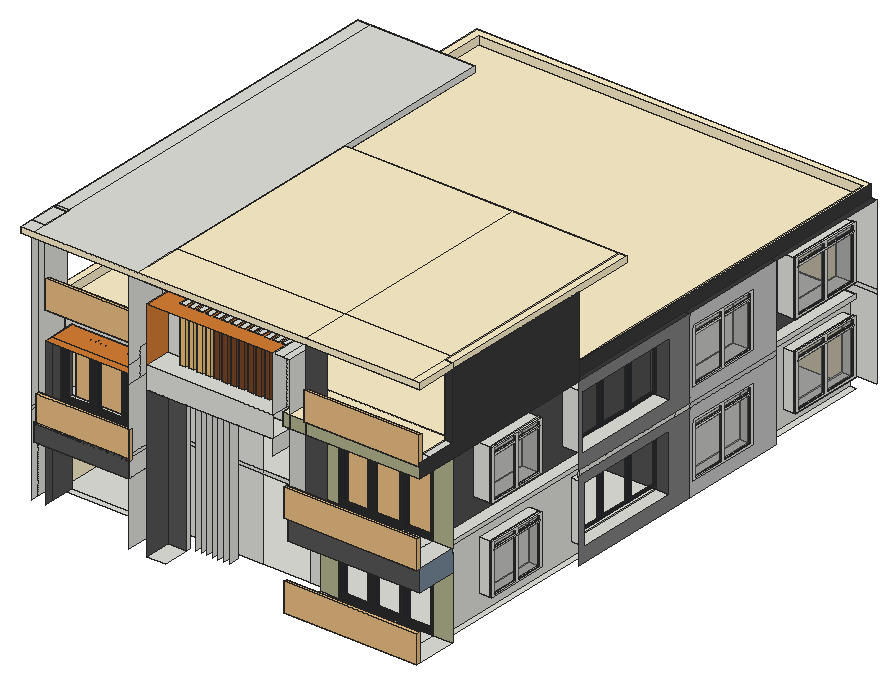
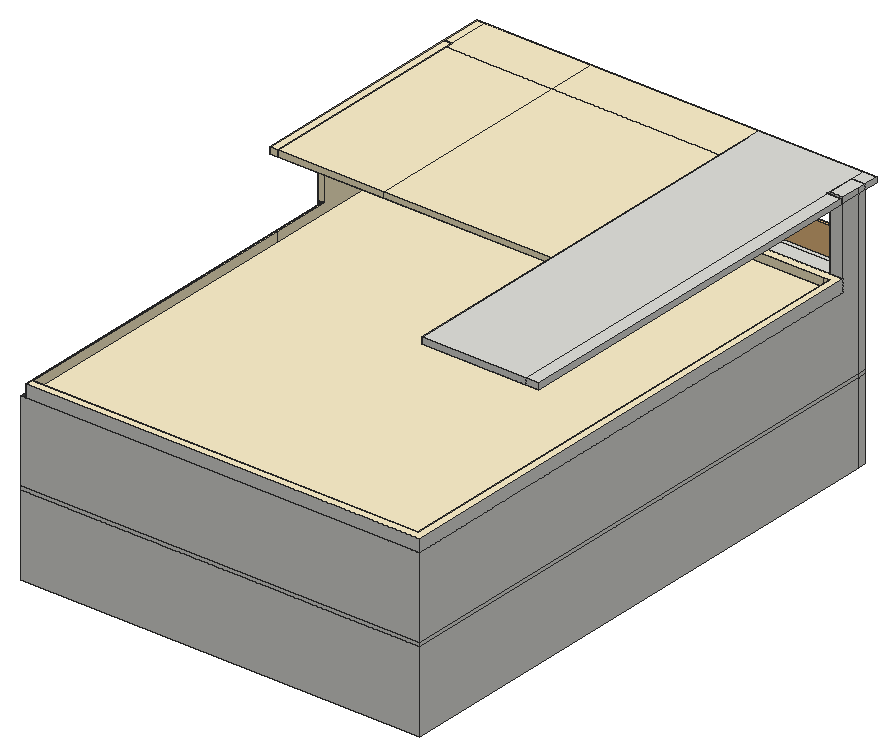
# SketchUp Ruby script. Lengths in inches.
U = 1.inch
M = Sketchup.active_model
def pt(a) = Geom::Point3d.new(a.map { |v| v * U })
def face(e, loops, mat)
  f = e.add_face(loops[0].map { |a| pt(a) })
  loops[1..].each { |l| e.add_face(l.map { |a| pt(a) }).erase! }
  f.material = f.back_material = mat if mat
  f
end
# faces: each face lists its corners as indices into pts; further lists are holes
def faces(e, pts, list, mat = nil) = list.each { |f| face(e, (f[0].is_a?(Array) ? f : [f]).map { |l| l.map { |i| pts[i] } }, mat) }
# xy, xz, yz: faces in a plane at the given z, y or x. An outline is a flat list of corners, or four numbers for a rectangle; further outlines are holes
def ring(l) = l.size == 4 ? [[l[0], l[1]], [l[2], l[1]], [l[2], l[3]], [l[0], l[3]]] : l.each_slice(2).to_a
def flat(e, list, mat, &to3) = list.each { |f| face(e, (f[0].is_a?(Array) ? f : [f]).map { |l| ring(l).map { |u, v| to3.(u, v) } }, mat) }
def xy(e, z, list, mat = nil) = flat(e, list, mat) { |x, y| [x, y, z] }
def xz(e, y, list, mat = nil) = flat(e, list, mat) { |x, z| [x, y, z] }
def yz(e, x, list, mat = nil) = flat(e, list, mat) { |y, z| [x, y, z] }
def lines(e, pts, list) = list.each { |a, b| e.add_line(pt(pts[a]), pt(pts[b])) }
# prism: a flat outline (further loops are holes) pulled along v
def prism(e, loops, v, mat = nil)
  f = face(e, loops, mat); d = Geom::Vector3d.new(v.map { |x| x * U })
  f.pushpull(f.normal.samedirection?(d) ? d.length : -d.length)
end
def box(e, o, s, mat = nil) = prism(e, [[o, [o[0] + s[0], o[1], o[2]], [o[0] + s[0], o[1] + s[1], o[2]], [o[0], o[1] + s[1], o[2]]]], [0, 0, s[2]], mat)
def at(x, y, z, deg = 0) = Geom::Transformation.translation(pt([x, y, z])) * Geom::Transformation.rotation(ORIGIN, Z_AXIS, deg.degrees)
def axes(o, x, y, z) = Geom::Transformation.new([*x, 0, *y, 0, *z, 0, *pt(o).to_a, 1])
def part(name) = M.definitions.add(name)
# library, detail: a bought-in or finely detailed component or shape, given as its bounding box
def library(name, o, s) = part(name).tap { |d| box(d.entities, o, s) }
def detail(e, o, s) = box(e.add_group.entities, o, s)
def put(e, d, t, mat = nil) = e.add_instance(d, t).tap { |i| i.material = mat if mat }
def group(e, t, mat = nil) = e.add_group.tap { |g| g.transformation = t; g.material = mat if mat }.entities
root = M.entities
M.materials.add("Wine2").color = [0, 0, 0]
M.materials["Wine2"].alpha = 0
M.materials.add("[0110_LightSlateGray]").color = [119, 136, 153]
M.materials.add("[0130_Gainsboro]").color = [39, 45, 50]
M.materials.add("[0133_Gray]").color = [128, 128, 128]
M.materials.add("[0135_DarkGray]1").color = [81, 81, 81]
M.materials.add("[Color D01]").color = [255, 242, 204]
M.materials.add("[Color E01]").color = [178, 178, 142]
M.materials.add("[Color M02]").color = [198, 198, 198]
M.materials.add("[Color M06]").color = [86, 86, 86]
M.materials.add("[Color M07]").color = [58, 58, 58]
M.materials.add("[Translucent Glass Gray]").color = [128, 128, 128]
M.materials["[Translucent Glass Gray]"].alpha = 0.5
M.materials.add("[Wood Bamboo]").color = [214, 127, 52]
M.materials.add("[Wood OSB]").color = [240, 195, 122]
M.materials.add("[Wood Veneer 01]").color = [120, 70, 37]
c1 = part("Framed glazing panel")
xy(c1.entities,0,[[0,-0.98,43.07,0],[0,0,43.07,1.4]],"[0130_Gainsboro]")
xy(c1.entities,0.3,[[0.3,-1.43,42.77,-0.98]],"[0130_Gainsboro]")
xy(c1.entities,2.95,[[2.95,-1.43,40.12,-0.63],[2.95,-0.63,40.12,0],[2.95,0,40.12,0.64],[2.95,0.64,40.12,1.4]],"[0130_Gainsboro]")
xy(c1.entities,3.54,[[3.54,-0.63,39.53,0],[3.54,0,39.53,0.64]],"[0130_Gainsboro]")
xy(c1.entities,111.8125,[[3.54,-0.63,39.53,0],[3.54,0,39.53,0.64]],"[0130_Gainsboro]")
xy(c1.entities,112.4,[[2.95,-1.43,40.12,-0.63],[2.95,-0.63,40.12,0],[2.95,0,40.12,0.64],[2.95,0.64,40.12,1.4]],"[0130_Gainsboro]")
xy(c1.entities,115.05,[[0.3,-1.43,42.77,-0.98]],"[0130_Gainsboro]")
xy(c1.entities,115.35,[[0,-0.98,43.07,0],[0,0,43.07,1.4]],"[0130_Gainsboro]")
xz(c1.entities,-1.43,[[[0.3,0.3,42.77,115.05],[2.95,2.95,40.12,112.4]]],"[0130_Gainsboro]")
xz(c1.entities,-0.98,[[[0,0,43.07,115.35],[0.3,0.3,42.77,115.05]]],"[0130_Gainsboro]")
xz(c1.entities,-0.63,[[[2.95,2.95,40.12,112.4],[3.54,3.54,39.53,111.8125]]],"[0130_Gainsboro]")
xz(c1.entities,0,[[3.54,3.54,39.53,111.8125]],"Wine2")
xz(c1.entities,0,[[[0,0,43.07,115.35],[2.95,2.95,40.12,112.4]],[[2.95,2.95,40.12,112.4],[3.54,3.54,39.53,111.8125]]],"[0130_Gainsboro]")
xz(c1.entities,0.64,[[[2.95,2.95,40.12,112.4],[3.54,3.54,39.53,111.8125]]],"[0130_Gainsboro]")
xz(c1.entities,1.4,[[[0,0,43.07,115.35],[2.95,2.95,40.12,112.4]]],"[0130_Gainsboro]")
yz(c1.entities,0,[[-0.98,0,0,115.35],[0,0,1.4,115.35]],"[0130_Gainsboro]")
yz(c1.entities,0.3,[[-1.43,0.3,-0.98,115.05]],"[0130_Gainsboro]")
yz(c1.entities,2.95,[[-1.43,2.95,-0.63,112.4],[-0.63,2.95,0,112.4],[0,2.95,0.64,112.4],[0.64,2.95,1.4,112.4]],"[0130_Gainsboro]")
yz(c1.entities,3.54,[[-0.63,3.54,0,111.8125],[0,3.54,0.64,111.8125]],"[0130_Gainsboro]")
yz(c1.entities,39.53,[[-0.63,3.54,0,111.8125],[0,3.54,0.64,111.8125]],"[0130_Gainsboro]")
yz(c1.entities,40.12,[[-1.43,2.95,-0.63,112.4],[-0.63,2.95,0,112.4],[0,2.95,0.64,112.4],[0.64,2.95,1.4,112.4]],"[0130_Gainsboro]")
yz(c1.entities,42.77,[[-1.43,0.3,-0.98,115.05]],"[0130_Gainsboro]")
yz(c1.entities,43.07,[[-0.98,0,0,115.35],[0,0,1.4,115.35]],"[0130_Gainsboro]")
c2 = part("Glazing assembly")
put(c2.entities,c1,axes([90.57,1.43,0],[1.05148,0,0],[0,1,0],[0,0,1]))
put(c2.entities,c1,axes([0,1.43,0],[1.05148,0,0],[0,1,0],[0,0,1]))
put(c2.entities,c1,axes([45.29,1.43,0],[1.05148,0,0],[0,1,0],[0,0,1]))
c3 = library("Glass Railing",[0,0,0],[139.5,4.76,42])
c4 = part("Group\#3")
xy(c4.entities,0,[[0,0,32.48,1.97]])
xy(c4.entities,0.98,[[0.98,0,31.5,0.98],[0.98,0.98,31.5,1.97]])
xy(c4.entities,8.86,[[0.98,0,31.5,0.98],[0.98,0.98,31.5,1.97]])
xy(c4.entities,9.84,[[0,0,32.48,1.97]])
xz(c4.entities,0,[[[0,0,32.48,9.84],[0.98,0.98,31.5,8.86]]])
xz(c4.entities,0.98,[[0.98,0.98,31.5,8.86]],"[Translucent Glass Gray]")
xz(c4.entities,1.97,[[[0,0,32.48,9.84],[0.98,0.98,31.5,8.86]]])
yz(c4.entities,0,[[0,0,1.97,9.84]])
yz(c4.entities,0.98,[[0,0.98,0.98,8.86],[0.98,0.98,1.97,8.86]])
yz(c4.entities,31.5,[[0,0.98,0.98,8.86],[0.98,0.98,1.97,8.86]])
yz(c4.entities,32.48,[[0,0,1.97,9.84]])
c5 = part("Group\#4")
xy(c5.entities,0,[[0,0,32.48,1.97]])
xy(c5.entities,0.98,[[0.98,0,31.5,0.98],[0.98,0.98,31.5,1.97]])
xy(c5.entities,71.85,[[0.98,0,31.5,0.98],[0.98,0.98,31.5,1.97]])
xy(c5.entities,72.83,[[0,0,32.48,1.97]])
xz(c5.entities,0,[[[0,0,32.48,72.83],[0.98,0.98,31.5,71.85]]])
xz(c5.entities,0.98,[[0.98,0.98,31.5,71.85]],"[Translucent Glass Gray]")
xz(c5.entities,1.97,[[[0,0,32.48,72.83],[0.98,0.98,31.5,71.85]]])
yz(c5.entities,0,[[0,0,1.97,72.83]])
yz(c5.entities,0.98,[[0,0.98,0.98,71.85],[0.98,0.98,1.97,71.85]])
yz(c5.entities,31.5,[[0,0.98,0.98,71.85],[0.98,0.98,1.97,71.85]])
yz(c5.entities,32.48,[[0,0,1.97,72.83]])
c6 = part("FIXED+GLASS+WINDOW+WITH+TRANSOM")
g1 = group(c6.entities,at(0,0,0))
xy(g1,0,[[0,0,70.86,3.9375]])
xy(g1,1.97,[[1.97,0,34.45,0.98],[36.42,0,68.9,3.9375],[1.97,2.95,34.45,3.9375]])
xy(g1,86.61,[[1.97,0,34.45,3.9375],[34.45,0,36.42,3.9375],[36.42,0,68.9,3.9375]])
xy(g1,88.58,[[0,0,70.86,3.9375]])
xz(g1,0,[[[0,0,70.86,88.58],[1.97,1.97,34.45,86.61],[36.42,1.97,68.9,86.61]]])
xz(g1,3.9375,[[[0,0,70.86,88.58],[1.97,1.97,34.45,86.61],[36.42,1.97,68.9,86.61]]])
yz(g1,0,[[0,0,3.9375,88.58]])
yz(g1,1.97,[[0,1.97,3.9375,74.8],[0,76.77,3.9375,86.61]])
yz(g1,34.45,[[0,1.97,3.9375,86.61]])
yz(g1,36.42,[[0,1.97,3.9375,86.61]])
yz(g1,68.9,[[0,1.97,3.9375,86.61]])
yz(g1,70.86,[[0,0,3.9375,88.58]])
g2 = group(g1,at(1.97,0,74.8))
box(g2,[0,0,0],[66.93,3.9375,1.97])
put(g1,c4,at(1.97,0.98,76.77))
put(g1,c4,at(36.42,0.98,76.77))
put(g1,c5,at(1.97,0.98,1.97))
put(g1,c5,at(36.42,0.98,1.97))
c7 = library("Group5_1",[-7.56,-66.38,0.11],[6.33,135.04,120.95])
xy(root,1007.625,[[326.68,240.0625,354.04,279.375],[536.21,240.3125,563.32,301.625],[563.32,240.3125,704.2,310.82],[704.2,240.3125,733.4375,301.625],[157.82,301.625,298.7,310.82],
  [146.57,310.82,713.5,1067.8],[713.5,310.82,721.74,1067.8]])
xy(root,1027.38,[[713.5,750.25,733.4375,861.32]])
xy(root,1029.41,[[631.25,546.17,713.5,704.54],[713.5,546.17,733.4375,704.54]])
xy(root,1032.83,[[713.5,942.08,733.4375,1053.14]])
xy(root,1036.03,[[713.5,375.23,733.4375,467.6]])
xy(root,1101.6875,[[563.32,301.625,704.2,310.82]])
xy(root,1101.6875,[[157.82,240.3125,298.7,273.3125],[536.21,240.3125,733.4375,301.625],[157.82,273.3125,298.7,310.82]],"[Wood Bamboo]")
xy(root,1108.63,[[713.5,750.25,733.4375,861.32]])
xy(root,1110.53,[[713.5,375.23,733.4375,467.6]])
xy(root,1114.08,[[713.5,942.08,733.4375,1053.14]])
xy(root,1114.73,[[631.25,546.17,713.5,704.54],[713.5,546.17,733.4375,704.54]])
xy(root,1127.625,[[157.82,240.3125,298.7,273.3125],[157.82,273.3125,298.7,301.625],[713.5,310.82,721.74,1067.8]])
xy(root,1127.625,[[146.57,310.82,713.5,1067.8]],"[Color D01]")
xy(root,1133.625,[[539.29,240.0625,563.32,240.3125],[536.21,240.3125,539.29,240.3125,539.29,279.375,563.32,279.375,563.32,301.625,536.21,301.625],[539.29,240.3125,563.32,279.375],[563.32,240.3125,704.2,310.82],[704.2,240.3125,733.4375,301.625],
  [157.82,301.625,298.7,310.82],[146.57,310.82,704.2,1067.8],[704.2,310.82,721.74,1067.8]])
xy(root,1153.38,[[704.2,750.25,733.4375,861.32]])
xy(root,1155.17,[[631.25,541.94,733.4375,706.32]])
xy(root,1158.83,[[704.2,942.08,733.4375,1053.14]])
xy(root,1162.03,[[704.2,375.23,733.4375,467.6]])
xy(root,1208.73,[[442.42,279.375,514.85,310.82]])
xy(root,1227.6875,[[563.32,301.625,704.2,310.82]])
xy(root,1227.6875,[[157.82,261.5,298.7,273.3125],[157.82,273.3125,298.7,310.82]],"[Wood Bamboo]")
xy(root,1230.97,[[326.68,240.0625,354.04,279.375],[354.04,240.0625,354.04,285.875,360.09,285.875,360.09,301.625,362.47,301.625,362.47,285.875,368.53,285.875,368.53,301.625,370.91,301.625,370.91,285.875,376.96,285.875,376.96,301.625,379.35,301.625,379.35,285.875,385.4,285.875,385.4,301.625,387.79,301.625,387.79,285.875,393.84,285.875,393.84,301.625,396.22,301.625,396.22,285.875,402.28,285.875,402.28,301.625,404.66,301.625,404.66,285.875,410.71,285.875,410.71,301.625,413.1,301.625,413.1,285.875,419.15,285.875,419.15,301.625,423.66,301.625,423.66,240.0625],[423.66,240.0625,514.85,279.375]])
xy(root,1234.63,[[704.2,750.25,733.4375,861.32]])
xy(root,1236.53,[[704.2,375.23,733.4375,467.6]])
xy(root,1237.73,[[631.25,541.94,733.4375,706.32]])
xy(root,1240.08,[[704.2,942.08,733.4375,1053.14]])
xy(root,1253.625,[[529.32,240.3125,536.21,301.625],[536.21,240.3125,733.4375,301.625],[[137.375,301.625,733.4375,301.625,733.4375,537.75,725.5,537.75,725.5,1091.875,137.375,1091.875],[146.57,310.82,704.2,1067.8]]])
xy(root,1253.625,[[725.5,537.75,733.4375,744.22],[725.5,744.22,733.4375,904.3],[725.5,904.3,733.4375,1091.875]],"[Color M07]")
xy(root,1259.625,[[148.92,313.17,721.89,1080.33]],"[Color D01]")
xy(root,1263.23,[[326.68,240.0625,514.85,240.0625,514.85,264.875,507.3125,264.875,507.3125,279.375,503.22,279.375,503.22,264.875,494.6875,264.875,494.6875,279.375,490.59,279.375,490.59,264.875,482.0625,264.875,482.0625,279.375,477.97,279.375,477.97,264.875,469.4375,264.875,469.4375,279.375,465.34,279.375,465.34,264.875,456.8125,264.875,456.8125,279.375,452.72,279.375,452.72,264.875,444.1875,264.875,444.1875,279.375,440.09,279.375,440.09,264.875,431.5625,264.875,431.5625,279.375,427.47,279.375,427.47,264.875,418.9375,264.875,418.9375,279.375,414.84,279.375,414.84,264.875,406.3125,264.875,406.3125,279.375,402.22,279.375,402.22,264.875,393.6875,264.875,393.6875,279.375,389.59,279.375,389.59,264.875,381.0625,264.875,381.0625,279.375,376.97,279.375,376.97,264.875,368.4375,264.875,368.4375,279.375,364.34,279.375,364.34,264.875,355.8125,264.875,355.8125,279.375,326.68,279.375]])
xy(root,1269.0625,[[157.51,261.5,298.7,273.3125],[157.51,273.3125,298.7,301.625]])
xy(root,1272.5,[[529.32,240.3125,721.89,240.3125,721.89,313.17,148.92,313.17,148.92,1080.33,721.89,1080.33,721.89,537.75,725.5,537.75,725.5,1091.875,137.375,1091.875,137.375,301.625,529.32,301.625]],"[Color D01]")
xy(root,1275.0625,[[721.89,240.3125,733.4375,258.53],[721.89,258.53,733.4375,301.625]])
xy(root,1345.48,[[514.85,240.0625,529.32,279.375],[529.32,240.0625,539.29,279.375],[355.8125,264.875,364.34,279.375],[368.4375,264.875,376.97,279.375],[381.0625,264.875,389.59,279.375],
  [393.6875,264.875,402.22,279.375],[406.3125,264.875,414.84,279.375],[418.9375,264.875,427.47,279.375],[431.5625,264.875,440.09,279.375],[444.1875,264.875,452.72,279.375],
  [456.8125,264.875,465.34,279.375],[469.4375,264.875,477.97,279.375],[482.0625,264.875,490.59,279.375],[494.6875,264.875,503.22,279.375],[507.3125,264.875,514.85,279.375]])
xy(root,1345.48,[[326.68,240.0625,326.68,279.375,355.8125,279.375,355.8125,264.875,364.34,264.875,364.34,279.375,368.4375,279.375,368.4375,264.875,376.97,264.875,376.97,279.375,381.0625,279.375,381.0625,264.875,389.59,264.875,389.59,279.375,393.6875,279.375,393.6875,264.875,402.22,264.875,402.22,279.375,406.3125,279.375,406.3125,264.875,414.84,264.875,414.84,279.375,418.9375,279.375,418.9375,264.875,427.47,264.875,427.47,279.375,431.5625,279.375,431.5625,264.875,440.09,264.875,440.09,279.375,444.1875,279.375,444.1875,264.875,452.72,264.875,452.72,279.375,456.8125,279.375,456.8125,264.875,465.34,264.875,465.34,279.375,469.4375,279.375,469.4375,264.875,477.97,264.875,477.97,279.375,482.0625,279.375,482.0625,264.875,490.59,264.875,490.59,279.375,494.6875,279.375,494.6875,264.875,503.22,264.875,503.22,279.375,507.3125,279.375,507.3125,264.875,514.85,264.875,514.85,240.0625]],"[Wood Bamboo]")
xy(root,1373.625,[[298.7,240.0625,312.6875,261.5],[312.6875,240.0625,312.6875,301.625,529.32,301.625,529.32,279.375,326.68,279.375,326.68,240.0625],[326.68,240.0625,563.32,279.375],[137.375,261.5,157.51,301.625],[298.7,261.5,312.6875,301.625],
  [298.7,301.625,312.6875,306.6875]])
xy(root,1373.625,[[721.89,301.625,733.4375,537.75],[721.89,537.75,733.4375,626.85]],"[Color D01]")
xy(root,1373.625,[[137.375,240.0625,137.375,261.5,157.51,261.5,157.51,306.6875,137.375,306.6875,137.375,869,312.6875,869,312.6875,306.6875,298.7,306.6875,298.7,240.0625],[563.32,240.0625,563.32,279.375,529.32,279.375,529.32,301.625,312.6875,301.625,312.6875,626.85,721.89,626.85,721.89,301.625,733.4375,301.625,733.4375,240.0625]],"[Color E01]")
xy(root,1382.3125,[[137.375,240.0625,157.51,261.5],[157.51,240.0625,312.6875,869],[137.375,261.5,157.51,301.625],[137.375,306.6875,157.51,869]])
xy(root,1382.3125,[[312.6875,240.0625,563.32,313.17],[563.32,240.0625,721.89,313.17],[721.89,240.0625,733.4375,301.625],[721.89,301.625,733.4375,626.85],[312.6875,313.17,563.32,626.85],
  [563.32,313.17,721.89,626.85]],"[Color D01]")
xz(root,240.0625,[[326.68,1230.97,514.85,1263.23]])
xz(root,240.0625,[[137.375,1373.625,733.4375,1382.3125]],"[Color D01]")
xz(root,240.3125,[[529.32,1253.625,733.4375,1253.625,733.4375,1275.0625,721.89,1275.0625,721.89,1272.5,529.32,1272.5]],"[Color E01]")
xz(root,240.3125,[[157.82,1101.6875,298.7,1127.625],[536.21,1101.6875,733.4375,1133.625]],"[Color M06]")
xz(root,261.5,[[137.375,1373.625,157.51,1382.3125]])
xz(root,264.875,[[355.8125,1263.23,364.34,1345.48],[368.4375,1263.23,376.97,1345.48],[381.0625,1263.23,389.59,1345.48],[393.6875,1263.23,402.22,1345.48]],"[Wood OSB]")
xz(root,264.875,[[406.3125,1263.23,414.84,1345.48],[418.9375,1263.23,427.47,1345.48],[431.5625,1263.23,440.09,1345.48],[444.1875,1263.23,452.72,1345.48],[456.8125,1263.23,465.34,1345.48],
  [469.4375,1263.23,477.97,1345.48],[482.0625,1263.23,490.59,1345.48],[494.6875,1263.23,503.22,1345.48],[507.3125,1263.23,514.85,1345.48]],"[Wood Veneer 01]")
xz(root,273.3125,[[157.82,1101.6875,298.7,1127.625]])
xz(root,279.375,[[[539.29,1133.625,539.29,1263.23,541.09,1263.23,541.09,1345.48,529.32,1345.48,529.32,1373.625,563.32,1373.625,563.32,1133.625],[545.1875,1263.23,553.72,1345.48]],[326.68,1263.23,355.8125,1345.48],[364.34,1263.23,368.4375,1345.48],[376.97,1263.23,381.0625,1345.48],[389.59,1263.23,393.6875,1345.48],
  [402.22,1263.23,406.3125,1345.48],[414.84,1263.23,418.9375,1345.48],[427.47,1263.23,431.5625,1345.48],[440.09,1263.23,444.1875,1345.48],[452.72,1263.23,456.8125,1345.48],
  [465.34,1263.23,469.4375,1345.48],[477.97,1263.23,482.0625,1345.48],[490.59,1263.23,494.6875,1345.48],[503.22,1263.23,507.3125,1345.48],[514.85,1263.23,515.84,1345.48],
  [519.9375,1263.23,528.47,1345.48],[532.5625,1263.23,539.29,1345.48],[539.29,1263.23,541.09,1345.48],[545.1875,1263.23,553.72,1345.48],[326.68,1345.48,529.32,1373.625]])
xz(root,279.375,[[326.68,1007.625,354.04,1230.97]],"[Color M06]")
xz(root,301.625,[[157.82,1127.625,298.7,1133.625],[137.375,1253.625,157.51,1272.5],[157.51,1253.625,298.7,1269.0625],[298.7,1253.625,529.32,1272.5],[157.51,1269.0625,298.7,1272.5],
  [137.375,1272.5,157.51,1373.625],[298.7,1272.5,529.32,1373.625],[137.375,1373.625,157.51,1382.3125]])
xz(root,301.625,[[721.89,1373.625,733.4375,1382.3125]],"[Color D01]")
xz(root,301.625,[[536.21,1007.625,563.32,1101.6875],[704.2,1007.625,733.4375,1101.6875],[536.21,1133.625,563.32,1133.625,563.32,1227.6875,704.2,1227.6875,704.2,1133.625,733.4375,1133.625,733.4375,1253.625,536.21,1253.625]],"[Color E01]")
xz(root,301.625,[[721.89,1275.0625,733.4375,1373.625]],"[Color M07]")
xz(root,306.6875,[[137.375,1373.625,157.51,1382.3125]])
xz(root,310.82,[[146.57,1007.625,146.57,1127.625,442.42,1127.625,442.42,1007.625,298.7,1007.625,298.7,1101.6875,157.82,1101.6875,157.82,1007.625],[514.85,1007.625,514.85,1127.625,713.5,1127.625,713.5,1007.625,704.2,1007.625,704.2,1101.6875,563.32,1101.6875,563.32,1007.625],[146.57,1127.625,442.42,1133.625],[442.42,1127.625,514.85,1133.625],[514.85,1127.625,721.74,1133.625],
  [146.57,1133.625,146.57,1253.625,704.2,1253.625,704.2,1227.6875,563.32,1227.6875,563.32,1133.625,514.85,1133.625,514.85,1208.73,442.42,1208.73,442.42,1133.625,298.7,1133.625,298.7,1227.6875,157.82,1227.6875,157.82,1133.625]])
xz(root,313.17,[[148.92,1259.625,157.51,1272.5],[157.51,1259.625,298.7,1272.5],[298.7,1259.625,529.32,1272.5],[529.32,1259.625,721.89,1272.5]],"[Color D01]")
xz(root,375.23,[[713.5,1036.03,733.4375,1110.53],[704.2,1162.03,733.4375,1236.53]])
xz(root,467.6,[[713.5,1036.03,733.4375,1110.53],[704.2,1162.03,733.4375,1236.53]])
xz(root,537.75,[[721.89,1272.5,733.4375,1373.625]],"[Color D01]")
xz(root,537.75,[[725.5,1253.625,733.4375,1272.5]],"[Color M07]")
xz(root,541.94,[[631.25,1155.17,733.4375,1237.73]])
xz(root,546.17,[[631.25,1029.41,713.5,1114.73],[713.5,1029.41,733.4375,1114.73]])
xz(root,626.85,[[312.6875,1373.625,563.32,1382.3125],[563.32,1373.625,721.89,1382.3125],[721.89,1373.625,733.4375,1382.3125]],"[Color D01]")
xz(root,704.54,[[631.25,1029.41,713.5,1114.73],[713.5,1029.41,733.4375,1114.73]],"[0135_DarkGray]1")
xz(root,706.32,[[631.25,1155.17,733.4375,1237.73]],"[0135_DarkGray]1")
xz(root,750.25,[[713.5,1027.38,733.4375,1108.63],[704.2,1153.38,733.4375,1234.63]])
xz(root,861.32,[[713.5,1027.38,733.4375,1108.63],[704.2,1153.38,733.4375,1234.63]])
xz(root,869,[[137.375,1373.625,157.51,1382.3125],[157.51,1373.625,312.6875,1382.3125]])
xz(root,942.08,[[713.5,1032.83,733.4375,1114.08],[704.2,1158.83,733.4375,1240.08]])
xz(root,1053.14,[[713.5,1032.83,733.4375,1114.08],[704.2,1158.83,733.4375,1240.08]])
xz(root,1067.8,[[146.57,1127.625,721.74,1133.625]])
xz(root,1067.8,[[146.57,1007.625,713.5,1127.625],[146.57,1133.625,704.2,1253.625]],"[Color D01]")
xz(root,1080.33,[[148.92,1259.625,721.89,1272.5]],"[Color D01]")
xz(root,1091.875,[[137.375,1007.625,733.4375,1127.625],[137.375,1127.625,733.4375,1133.625],[137.375,1133.625,733.4375,1253.625],[137.375,1253.625,725.5,1272.5]])
yz(root,137.375,[[261.5,1007.625,273.3125,1127.625],[273.3125,1007.625,1091.875,1127.625],[261.5,1127.625,273.3125,1133.625],[273.3125,1127.625,1091.875,1133.625],[261.5,1133.625,273.3125,1373.625],
  [273.3125,1133.625,273.3125,1373.625,301.625,1373.625,301.625,1253.625,1091.875,1253.625,1091.875,1133.625],[301.625,1253.625,1091.875,1272.5],[240.0625,1373.625,261.5,1382.3125],[261.5,1373.625,273.3125,1382.3125],[273.3125,1373.625,301.625,1382.3125],
  [306.6875,1373.625,869,1382.3125]])
yz(root,146.57,[[310.82,1127.625,1067.8,1133.625]])
yz(root,146.57,[[310.82,1007.625,1067.8,1127.625],[310.82,1133.625,1067.8,1253.625]],"[Color D01]")
yz(root,148.92,[[313.17,1259.625,1080.33,1272.5]],"[Color D01]")
yz(root,157.51,[[261.5,1269.0625,301.625,1373.625],[261.5,1373.625,301.625,1382.3125],[301.625,1373.625,306.6875,1382.3125]])
yz(root,157.82,[[240.3125,1101.6875,261.5,1127.625],[261.5,1101.6875,273.3125,1127.625]])
yz(root,157.82,[[261.5,1007.625,273.3125,1101.6875],[273.3125,1007.625,310.82,1101.6875],[261.5,1127.625,273.3125,1133.625],[273.3125,1127.625,301.625,1133.625],[261.5,1133.625,273.3125,1227.6875],
  [273.3125,1133.625,310.82,1227.6875]],"[Color M06]")
yz(root,298.7,[[240.0625,1007.625,310.82,1101.6875],[240.0625,1101.6875,240.3125,1127.625],[240.3125,1101.6875,273.3125,1127.625],[240.0625,1127.625,301.625,1133.625],[240.0625,1133.625,310.82,1227.6875],
  [240.0625,1227.6875,261.5,1253.625],[261.5,1227.6875,273.3125,1269.0625],[240.0625,1253.625,240.0625,1373.625,301.625,1373.625,301.625,1269.0625,261.5,1269.0625,261.5,1253.625]])
yz(root,312.6875,[[261.5,1373.625,301.625,1382.3125],[301.625,1373.625,306.6875,1382.3125],[626.85,1373.625,869,1382.3125]])
yz(root,312.6875,[[306.6875,1373.625,313.17,1382.3125],[313.17,1373.625,626.85,1382.3125]],"[Color D01]")
yz(root,326.68,[[240.0625,1007.625,279.375,1230.97]],"[Color M06]")
yz(root,326.68,[[240.0625,1263.23,279.375,1345.48]],"[Wood Bamboo]")
yz(root,354.04,[[279.375,1007.625,285.875,1230.97]])
yz(root,355.8125,[[264.875,1263.23,279.375,1345.48]])
yz(root,362.47,[[285.875,1007.625,301.625,1230.97]])
yz(root,364.34,[[264.875,1263.23,279.375,1345.48]],"[Wood OSB]")
yz(root,368.4375,[[264.875,1263.23,279.375,1345.48]])
yz(root,370.91,[[285.875,1007.625,301.625,1230.97]])
yz(root,376.97,[[264.875,1263.23,279.375,1345.48]],"[Wood OSB]")
yz(root,379.35,[[285.875,1007.625,301.625,1230.97]])
yz(root,381.0625,[[264.875,1263.23,279.375,1345.48]])
yz(root,387.79,[[285.875,1007.625,301.625,1230.97]])
yz(root,389.59,[[264.875,1263.23,279.375,1345.48]],"[Wood OSB]")
yz(root,393.6875,[[264.875,1263.23,279.375,1345.48]])
yz(root,396.22,[[285.875,1007.625,301.625,1230.97]])
yz(root,402.22,[[264.875,1263.23,279.375,1345.48]],"[Wood OSB]")
yz(root,404.66,[[285.875,1007.625,301.625,1230.97]])
yz(root,406.3125,[[264.875,1263.23,279.375,1345.48]])
yz(root,413.1,[[285.875,1007.625,301.625,1230.97]])
yz(root,414.84,[[264.875,1263.23,279.375,1345.48]],"[Wood Veneer 01]")
yz(root,418.9375,[[264.875,1263.23,279.375,1345.48]])
yz(root,427.47,[[264.875,1263.23,279.375,1345.48]],"[Wood Veneer 01]")
yz(root,431.5625,[[264.875,1263.23,279.375,1345.48]])
yz(root,440.09,[[264.875,1263.23,279.375,1345.48]],"[Wood Veneer 01]")
yz(root,444.1875,[[264.875,1263.23,279.375,1345.48]])
yz(root,452.72,[[264.875,1263.23,279.375,1345.48]],"[Wood Veneer 01]")
yz(root,456.8125,[[264.875,1263.23,279.375,1345.48]])
yz(root,465.34,[[264.875,1263.23,279.375,1345.48]],"[Wood Veneer 01]")
yz(root,469.4375,[[264.875,1263.23,279.375,1345.48]])
yz(root,477.97,[[264.875,1263.23,279.375,1345.48]],"[Wood Veneer 01]")
yz(root,482.0625,[[264.875,1263.23,279.375,1345.48]])
yz(root,490.59,[[264.875,1263.23,279.375,1345.48]],"[Wood Veneer 01]")
yz(root,494.6875,[[264.875,1263.23,279.375,1345.48]])
yz(root,503.22,[[264.875,1263.23,279.375,1345.48]])
yz(root,507.3125,[[264.875,1263.23,279.375,1345.48]])
yz(root,514.85,[[240.0625,1208.73,279.375,1230.97],[240.0625,1263.23,264.875,1345.48],[264.875,1263.23,279.375,1345.48]])
yz(root,529.32,[[240.3125,1253.625,301.625,1272.5]])
yz(root,536.21,[[240.3125,1101.6875,301.625,1133.625]])
yz(root,539.29,[[240.0625,1133.625,279.375,1345.48]])
yz(root,563.32,[[301.625,1007.625,310.82,1101.6875],[301.625,1133.625,310.82,1227.6875]])
yz(root,563.32,[[240.0625,1133.625,279.375,1373.625]],"[Color M06]")
yz(root,631.25,[[541.94,1155.17,706.32,1237.73]])
yz(root,631.25,[[546.17,1029.41,704.54,1114.73]],"[0135_DarkGray]1")
yz(root,704.2,[[301.625,1007.625,310.82,1101.6875],[301.625,1133.625,310.82,1227.6875]])
yz(root,704.2,[[[310.82,1133.625,1067.8,1253.625],[750.25,1153.38,861.32,1234.63],[942.08,1158.83,1053.14,1240.08],[375.23,1162.03,467.6,1236.53]]],"[0135_DarkGray]1")
yz(root,713.5,[[[310.82,1007.625,1067.8,1127.625],[546.17,1029.41,704.54,1114.73],[750.25,1027.38,861.32,1108.63],[942.08,1032.83,1053.14,1114.08],[375.23,1036.03,467.6,1110.53]]])
yz(root,721.74,[[310.82,1127.625,1067.8,1133.625]])
yz(root,721.89,[[313.17,1259.625,313.17,1373.625,537.75,1373.625,537.75,1272.5,626.85,1272.5,626.85,1259.625],[626.85,1259.625,1080.33,1272.5],[240.3125,1272.5,258.53,1275.0625],[258.53,1272.5,301.625,1275.0625],[301.625,1272.5,313.17,1373.625],
  [301.625,1373.625,313.17,1382.3125],[313.17,1373.625,626.85,1382.3125]],"[Color D01]")
yz(root,725.5,[[537.75,1253.625,1091.875,1272.5]],"[Color M07]")
yz(root,733.4375,[[534.42,1127.625,537.75,1133.625],[537.75,1127.625,716.73,1133.625],[716.73,1127.625,744.22,1133.625]])
yz(root,733.4375,[[240.3125,1101.6875,301.625,1101.6875,301.625,1127.625,300.15,1127.625,300.15,1133.625,240.3125,1133.625]],"[0110_LightSlateGray]")
yz(root,733.4375,[[[537.75,1007.625,744.22,1127.625],[546.17,1029.41,704.54,1114.73]],[[537.75,1133.625,744.22,1253.625],[541.94,1155.17,706.32,1237.73]]],"[0133_Gray]")
yz(root,733.4375,[[240.0625,1373.625,301.625,1382.3125],[301.625,1373.625,626.85,1382.3125]],"[Color D01]")
yz(root,733.4375,[[[744.22,1007.625,904.3,1127.625],[750.25,1027.38,861.32,1108.63]],[744.22,1127.625,904.3,1133.625],[[744.22,1133.625,904.3,1253.625],[750.25,1153.38,861.32,1234.63]]],"[Color M02]")
yz(root,733.4375,[[240.3125,1253.625,537.75,1253.625,537.75,1373.625,301.625,1373.625,301.625,1275.0625,240.3125,1275.0625]],"[Color M07]")
p = [[733.4375,301.625,1127.625],[731.625,301.625,1127.625],[733.4375,300.15,1133.625],[563.32,313.17,1373.625],[563.32,313.17,1382.3125],[563.32,258.53,1259.625],
  [721.89,258.53,1259.625]]
lines(root,p,[[0,1],[1,2],[3,4],[5,6]])
put(root,c2,axes([563.32,312.95,1007.625],[1.03691,0,0],[0,-4,0],[0,0,0.80657]))
put(root,c3,axes([534.23,235.55,1007.625],[1.428,0,0],[0,1,0],[0,0,1]))
put(root,c6,axes([733.4375,750.25,1027.38],[0,1.56726,0],[-1,0,0],[0,0,0.91722]))
put(root,c2,axes([713.5,549.13,1033.77],[0,1.17066,0],[-1.13,0,0],[0,0,0.72061]))
put(root,c6,axes([733.4375,942.08,1034.15],[0,1.56726,0],[-1,0,0],[0,0,0.91722]))
put(root,c6,axes([733.4375,375.23,1036.03],[0,1.30355,0],[-1,0,0],[0,0,0.84102]))
put(root,c3,at(161,240.3125,1125.07))
put(root,c7,axes([230.04,309.6,1127.02],[0,-1,0],[1,0,0],[0,0,0.83156]))
put(root,c7,axes([635.54,309.6,1127.02],[0,-1,0],[1,0,0],[0,0,0.83156]))
put(root,c2,axes([157.82,301.625,1133.625],[1.03691,0,0],[0,-4,0],[0,0,0.80657]))
put(root,c2,axes([563.32,312.95,1133.625],[1.03691,0,0],[0,-4,0],[0,0,0.80657]))
put(root,c3,axes([534.23,235.55,1133.625],[1.428,0,0],[0,1,0],[0,0,1]))
put(root,c6,axes([733.4375,750.25,1153.38],[0,1.56726,0],[-1,0,0],[0,0,0.91722]))
put(root,c2,axes([713.5,549.13,1157.52],[0,1.17066,0],[-1.13,0,0],[0,0,0.72061]))
put(root,c6,axes([733.4375,942.08,1160.15],[0,1.56726,0],[-1,0,0],[0,0,0.91722]))
put(root,c6,axes([733.4375,375.23,1162.03],[0,1.30355,0],[-1,0,0],[0,0,0.84102]))
put(root,c3,at(157.51,261.5,1269.0625))
put(root,c3,axes([562.12,238.55,1271.49],[1.22808,0,0],[0,1,0],[0,0,1]))
